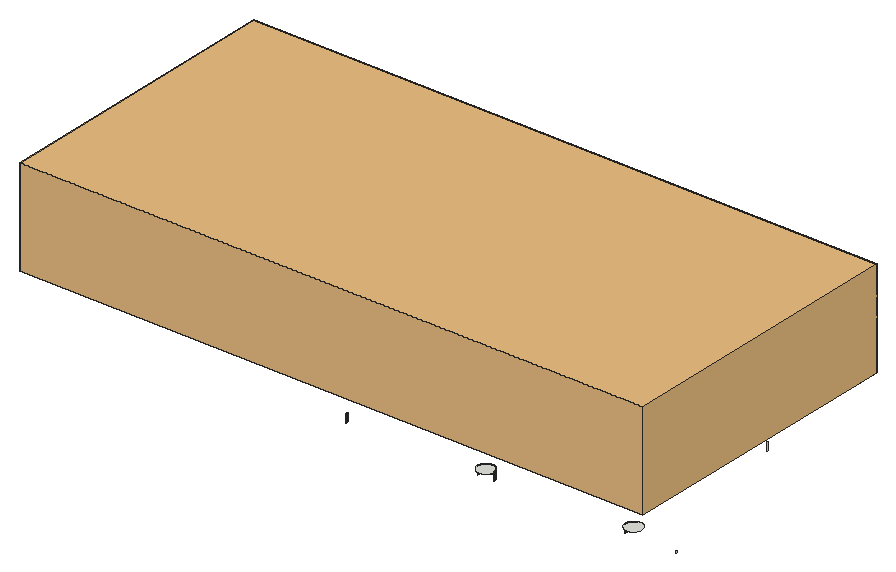
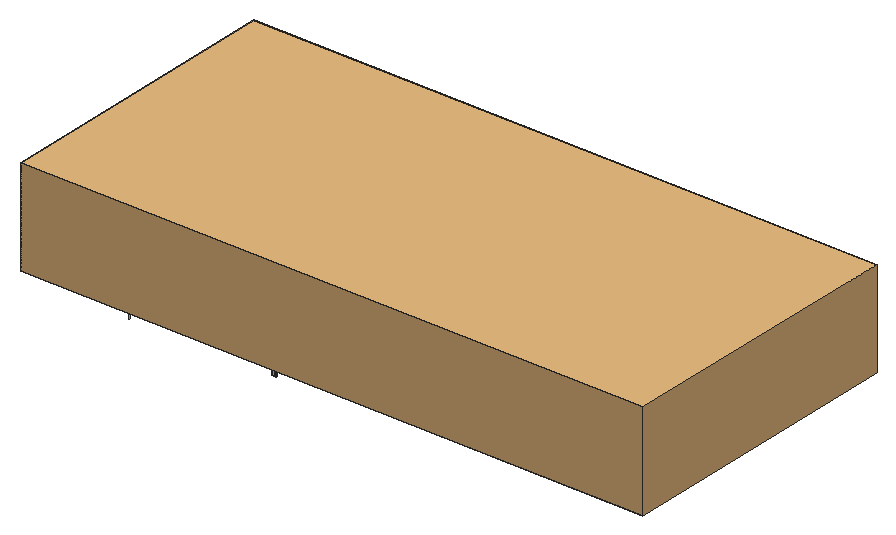
# SketchUp Ruby script. Lengths in inches.
U = 1.inch
M = Sketchup.active_model
def pt(a) = Geom::Point3d.new(a.map { |v| v * U })
def face(e, loops, mat)
  f = e.add_face(loops[0].map { |a| pt(a) })
  loops[1..].each { |l| e.add_face(l.map { |a| pt(a) }).erase! }
  f.material = f.back_material = mat if mat
  f
end
# faces: each face lists its corners as indices into pts; further lists are holes
def faces(e, pts, list, mat = nil) = list.each { |f| face(e, (f[0].is_a?(Array) ? f : [f]).map { |l| l.map { |i| pts[i] } }, mat) }
# xy, xz, yz: faces in a plane at the given z, y or x. An outline is a flat list of corners, or four numbers for a rectangle; further outlines are holes
def ring(l) = l.size == 4 ? [[l[0], l[1]], [l[2], l[1]], [l[2], l[3]], [l[0], l[3]]] : l.each_slice(2).to_a
def flat(e, list, mat, &to3) = list.each { |f| face(e, (f[0].is_a?(Array) ? f : [f]).map { |l| ring(l).map { |u, v| to3.(u, v) } }, mat) }
def xy(e, z, list, mat = nil) = flat(e, list, mat) { |x, y| [x, y, z] }
def xz(e, y, list, mat = nil) = flat(e, list, mat) { |x, z| [x, y, z] }
def yz(e, x, list, mat = nil) = flat(e, list, mat) { |y, z| [x, y, z] }
def lines(e, pts, list) = list.each { |a, b| e.add_line(pt(pts[a]), pt(pts[b])) }
# prism: a flat outline (further loops are holes) pulled along v
def prism(e, loops, v, mat = nil)
  f = face(e, loops, mat); d = Geom::Vector3d.new(v.map { |x| x * U })
  f.pushpull(f.normal.samedirection?(d) ? d.length : -d.length)
end
def box(e, o, s, mat = nil) = prism(e, [[o, [o[0] + s[0], o[1], o[2]], [o[0] + s[0], o[1] + s[1], o[2]], [o[0], o[1] + s[1], o[2]]]], [0, 0, s[2]], mat)
def at(x, y, z, deg = 0) = Geom::Transformation.translation(pt([x, y, z])) * Geom::Transformation.rotation(ORIGIN, Z_AXIS, deg.degrees)
def axes(o, x, y, z) = Geom::Transformation.new([*x, 0, *y, 0, *z, 0, *pt(o).to_a, 1])
def part(name) = M.definitions.add(name)
# library, detail: a bought-in or finely detailed component or shape, given as its bounding box
def library(name, o, s) = part(name).tap { |d| box(d.entities, o, s) }
def detail(e, o, s) = box(e.add_group.entities, o, s)
def put(e, d, t, mat = nil) = e.add_instance(d, t).tap { |i| i.material = mat if mat }
def group(e, t, mat = nil) = e.add_group.tap { |g| g.transformation = t; g.material = mat if mat }.entities
root = M.entities
M.materials.add("[Steel Brushed Stainless]1").color = [76, 76, 76]
c1 = library("Group\#19",[-3,0,0],[231,108,36])
xy(root,234,[[269.08,185,269,185.01,268.92,185.01,268.76,185.03,268.6875,185.04,268.61,185.06,268.53,185.08,268.46,185.09,268.38,185.11,268.3,185.14,268.23,185.16,268.16,185.1875,268.08,185.22,268.01,185.25,267.9375,185.28,267.87,185.3125,267.8,185.35,267.73,185.39,267.66,185.42,267.59,185.47,267.53,185.51,267.46,185.55,267.16,185.8,266.99,185.97,266.79,186.21,266.75,186.27,266.7,186.34,266.66,186.4,266.54,186.61,266.51,186.68,266.47,186.75,266.41,186.89,266.38,186.97,266.36,187.04,266.33,187.12,266.3125,187.19,266.29,187.27,266.27,187.34,266.26,187.42,266.24,187.5,266.23,187.58,266.22,187.65,266.21,187.73,266.21,187.81,266.2,187.89,266.2,188.125,266.21,188.2,266.21,188.28,266.22,188.36,266.23,188.4375,266.24,188.51,266.28,188.67,266.29,188.74,266.3125,188.82,266.34,188.9,266.36,188.97,266.39,189.04,266.42,189.12,266.51,189.33,266.59,189.47,266.625,189.54,266.67,189.61,266.71,189.67,266.75,189.74,267,190.04,267.17,190.21,267.41,190.41,267.47,190.45,267.54,190.5,267.6,190.54,267.81,190.66,267.88,190.69,267.95,190.73,268.09,190.79,268.17,190.82,268.24,190.84,268.32,190.87,268.39,190.89,268.47,190.91,268.54,190.93,268.62,190.94,268.7,190.96,268.78,190.97,268.85,190.98,268.93,190.99,269.01,190.99,269.09,191,269.32,191,269.4,190.99,269.48,190.99,269.64,190.97,269.71,190.96,269.87,190.92,269.94,190.91,270.02,190.89,270.1,190.86,270.17,190.84,270.24,190.8125,270.32,190.78,270.46,190.72,270.53,190.6875,270.6,190.65,270.67,190.61,270.74,190.58,270.81,190.53,270.87,190.49,270.9375,190.45,271.0625,190.35,271.12,190.3,271.24,190.2,271.41,190.03,271.61,189.79,271.65,189.73,271.7,189.66,271.74,189.6,271.86,189.39,271.89,189.32,271.93,189.25,271.99,189.11,272.02,189.03,272.04,188.96,272.07,188.88,272.09,188.81,272.11,188.73,272.13,188.66,272.14,188.58,272.16,188.5,272.17,188.42,272.18,188.35,272.1875,188.27,272.19,188.19,272.2,188.11,272.2,187.875,272.19,187.8,272.1875,187.72,272.18,187.64,272.17,187.5625,272.16,187.49,272.14,187.41,272.125,187.33,272.11,187.26,272.09,187.18,272.0625,187.1,272.04,187.03,272.01,186.96,271.98,186.88,271.89,186.67,271.81,186.53,271.78,186.46,271.73,186.39,271.69,186.33,271.65,186.26,271.4,185.96,271.23,185.79,270.99,185.59,270.93,185.55,270.86,185.5,270.8,185.46,270.59,185.34,270.52,185.31,270.45,185.27,270.31,185.21,270.23,185.18,270.16,185.16,270.08,185.13,270.01,185.11,269.93,185.09,269.86,185.07,269.78,185.06,269.7,185.04,269.55,185.02,269.47,185.01,269.39,185.01,269.3125,185],[323.875,185,323.8,185.01,323.72,185.01,323.64,185.02,323.5625,185.03,323.49,185.04,323.33,185.08,323.26,185.09,323.18,185.11,323.1,185.14,323.03,185.16,322.96,185.1875,322.88,185.22,322.74,185.28,322.67,185.3125,322.6,185.35,322.53,185.39,322.46,185.42,322.39,185.47,322.33,185.51,322.26,185.55,321.96,185.8,321.79,185.97,321.59,186.21,321.55,186.27,321.5,186.34,321.46,186.4,321.34,186.61,321.31,186.68,321.27,186.75,321.21,186.89,321.18,186.97,321.16,187.04,321.13,187.12,321.11,187.19,321.09,187.27,321.07,187.34,321.06,187.42,321.04,187.5,321.03,187.58,321.02,187.65,321.01,187.73,321.01,187.81,321,187.89,321,188.125,321.01,188.2,321.01,188.28,321.02,188.36,321.03,188.4375,321.04,188.51,321.08,188.67,321.09,188.74,321.11,188.82,321.14,188.9,321.16,188.97,321.1875,189.04,321.22,189.12,321.28,189.26,321.3125,189.33,321.35,189.4,321.39,189.47,321.42,189.54,321.47,189.61,321.51,189.67,321.55,189.74,321.8,190.04,321.97,190.21,322.21,190.41,322.27,190.45,322.34,190.5,322.4,190.54,322.61,190.66,322.68,190.69,322.75,190.73,322.89,190.79,322.97,190.82,323.04,190.84,323.12,190.87,323.19,190.89,323.27,190.91,323.34,190.93,323.42,190.94,323.5,190.96,323.58,190.97,323.65,190.98,323.73,190.99,323.81,190.99,323.89,191,324.125,191,324.2,190.99,324.28,190.99,324.36,190.98,324.4375,190.97,324.51,190.96,324.67,190.92,324.74,190.91,324.82,190.89,324.9,190.86,324.97,190.84,325.04,190.8125,325.12,190.78,325.26,190.72,325.33,190.6875,325.4,190.65,325.47,190.61,325.54,190.58,325.61,190.53,325.67,190.49,325.74,190.45,326.04,190.2,326.21,190.03,326.41,189.79,326.45,189.73,326.5,189.66,326.54,189.6,326.66,189.39,326.69,189.32,326.73,189.25,326.79,189.11,326.82,189.03,326.84,188.96,326.87,188.88,326.89,188.81,326.91,188.73,326.93,188.66,326.94,188.58,326.96,188.5,326.97,188.42,326.98,188.35,326.99,188.27,326.99,188.19,327,188.11,327,187.875,326.99,187.8,326.99,187.72,326.98,187.64,326.97,187.5625,326.96,187.49,326.92,187.33,326.91,187.26,326.89,187.18,326.86,187.1,326.84,187.03,326.8125,186.96,326.78,186.88,326.72,186.74,326.6875,186.67,326.65,186.6,326.61,186.53,326.58,186.46,326.53,186.39,326.49,186.33,326.45,186.26,326.2,185.96,326.03,185.79,325.79,185.59,325.73,185.55,325.66,185.5,325.6,185.46,325.39,185.34,325.32,185.31,325.25,185.27,325.11,185.21,325.03,185.18,324.96,185.16,324.88,185.13,324.81,185.11,324.73,185.09,324.66,185.07,324.58,185.06,324.5,185.04,324.42,185.03,324.35,185.02,324.27,185.01,324.19,185.01,324.11,185]])
xz(root,190.99,[[268.93,231,269.01,234],[269.4,231,269.48,234]])
xz(root,191,[[269.09,231,269.17,234],[269.17,231,269.25,234],[269.25,231,269.32,234]])
xz(root,251,[[269.08,231,269.15,234],[269.15,231,269.23,234],[269.23,231,269.3125,234]])
xz(root,251.01,[[268.92,231,269,234],[269.39,231,269.47,234]])
yz(root,217.39,[[188.19,231,188.27,234]])
yz(root,217.4,[[187.875,231,187.95,234],[187.95,231,188.03,234],[188.03,231,188.11,234]])
yz(root,266.2,[[187.89,231,187.97,234],[187.97,231,188.05,234],[188.05,231,188.125,234]])
yz(root,266.21,[[188.2,231,188.28,234]])
yz(root,272.2,[[187.875,231,187.95,234],[187.95,231,188.03,234],[188.03,231,188.11,234]])
yz(root,321,[[187.89,231,187.97,234],[187.97,231,188.05,234],[188.05,231,188.125,234]])
yz(root,321.01,[[188.2,231,188.28,234]])
yz(root,340,[[187.79,231,188,231.5]])
p = [[217.39,188.19,231],[217.4,188.11,231],[217.4,188.11,234],[217.39,188.19,234],[266.2,188.125,231],[266.21,188.2,231],
  [266.21,188.2,234],[266.2,188.125,234],[272.19,188.19,231],[272.2,188.11,231],[272.2,188.11,234],[272.19,188.19,234],
  [321,188.125,231],[321.01,188.2,231],[321.01,188.2,234],[321,188.125,234],[272.1875,188.27,231],[272.1875,188.27,234],
  [217.37,188.42,231],[217.38,188.35,231],[217.38,188.35,234],[217.37,188.42,234],[217.39,188.27,231],[217.39,188.27,234],
  [266.21,188.28,231],[266.22,188.36,231],[266.22,188.36,234],[266.21,188.28,234],[272.17,188.42,231],[272.18,188.35,231],
  [272.18,188.35,234],[272.17,188.42,234],[321.01,188.28,231],[321.02,188.36,231],[321.02,188.36,234],[321.01,188.28,234],
  [217.36,188.5,231],[217.36,188.5,234],[266.23,188.4375,231],[266.23,188.4375,234],[266.24,188.51,231],[266.24,188.51,234],
  [272.16,188.5,231],[272.16,188.5,234],[321.03,188.4375,231],[321.03,188.4375,234],[321.04,188.51,231],[321.04,188.51,234],
  [217.34,188.58,231],[217.34,188.58,234],[266.26,188.59,231],[266.26,188.59,234],[272.14,188.58,231],[272.14,188.58,234],
  [321.06,188.59,231],[321.06,188.59,234],[217.33,188.66,231],[217.33,188.66,234],[266.28,188.67,231],[266.28,188.67,234],
  [272.13,188.66,231],[272.13,188.66,234],[321.08,188.67,231],[321.08,188.67,234],[217.29,188.81,231],[217.31,188.73,231],
  [217.31,188.73,234],[217.29,188.81,234],[266.29,188.74,231],[266.29,188.74,234],[266.3125,188.82,231],[266.3125,188.82,234],
  [272.09,188.81,231],[272.11,188.73,231],[272.11,188.73,234],[272.09,188.81,234],[321.09,188.74,231],[321.09,188.74,234],
  [321.11,188.82,231],[321.11,188.82,234],[217.27,188.88,231],[217.27,188.88,234],[266.34,188.9,231],[266.34,188.9,234],
  [272.07,188.88,231],[272.07,188.88,234],[321.14,188.9,231],[321.14,188.9,234],[266.36,188.97,231],[266.36,188.97,234],
  [272.04,188.96,231],[272.04,188.96,234],[321.16,188.97,231],[321.16,188.97,234],[266.39,189.04,231],[266.39,189.04,234],
  [266.42,189.12,231],[266.42,189.12,234],[271.99,189.11,231],[272.02,189.03,231],[272.02,189.03,234],[271.99,189.11,234],
  [321.1875,189.04,231],[321.1875,189.04,234],[321.22,189.12,231],[321.22,189.12,234],[266.45,189.19,231],[266.45,189.19,234],
  [271.96,189.18,231],[271.96,189.18,234],[321.25,189.19,231],[321.25,189.19,234],[266.48,189.26,231],[266.48,189.26,234],
  [271.93,189.25,231],[271.93,189.25,234],[321.28,189.26,231],[321.28,189.26,234],[266.51,189.33,231],[266.51,189.33,234],
  [266.55,189.4,231],[266.55,189.4,234],[271.86,189.39,231],[271.89,189.32,231],[271.89,189.32,234],[271.86,189.39,234],
  [321.3125,189.33,231],[321.3125,189.33,234],[321.35,189.4,231],[321.35,189.4,234],[266.59,189.47,231],[266.59,189.47,234],
  [271.82,189.46,231],[271.82,189.46,234],[321.39,189.47,231],[321.39,189.47,234],[266.625,189.54,231],[266.625,189.54,234],
  [266.67,189.61,231],[266.67,189.61,234],[271.74,189.6,231],[271.78,189.53,231],[271.78,189.53,234],[271.74,189.6,234],
  [321.42,189.54,231],[321.42,189.54,234],[321.47,189.61,231],[321.47,189.61,234],[266.71,189.67,231],[266.71,189.67,234],
  [271.7,189.66,231],[271.7,189.66,234],[321.51,189.67,231],[321.51,189.67,234],[266.75,189.74,231],[266.75,189.74,234],
  [266.8,189.8,231],[266.8,189.8,234],[271.61,189.79,231],[271.65,189.73,231],[271.65,189.73,234],[271.61,189.79,234],
  [321.55,189.74,231],[321.55,189.74,234],[321.6,189.8,231],[321.6,189.8,234],[266.85,189.86,231],[266.85,189.86,234],
  [271.56,189.85,231],[271.56,189.85,234],[321.65,189.86,231],[321.65,189.86,234],[266.9,189.92,231],[266.9,189.92,234],
  [266.95,189.98,231],[266.95,189.98,234],[271.46,189.97,231],[271.51,189.91,231],[271.51,189.91,234],[271.46,189.97,234],
  [321.7,189.92,231],[321.7,189.92,234],[321.75,189.98,231],[321.75,189.98,234],[267,190.04,231],[267,190.04,234],
  [267.06,190.1,231],[267.06,190.1,234],[271.35,190.09,231],[271.41,190.03,231],[271.41,190.03,234],[271.35,190.09,234],
  [321.8,190.04,231],[321.8,190.04,234],[321.86,190.1,231],[321.86,190.1,234],[267.11,190.15,231],[267.11,190.15,234],
  [271.24,190.2,231],[271.3,190.14,231],[271.3,190.14,234],[271.24,190.2,234],[321.91,190.15,231],[321.91,190.15,234],
  [267.17,190.21,231],[267.17,190.21,234],[267.23,190.26,231],[267.23,190.26,234],[271.18,190.25,231],[271.18,190.25,234],
  [321.97,190.21,231],[321.97,190.21,234],[322.03,190.26,231],[322.03,190.26,234],[267.29,190.31,231],[267.29,190.31,234],
  [267.35,190.36,231],[267.35,190.36,234],[271.0625,190.35,231],[271.12,190.3,231],[271.12,190.3,234],[271.0625,190.35,234],
  [322.09,190.31,231],[322.09,190.31,234],[322.15,190.36,231],[322.15,190.36,234],[267.41,190.41,231],[267.41,190.41,234],
  [267.47,190.45,231],[267.47,190.45,234],[270.87,190.49,231],[270.9375,190.45,231],[270.9375,190.45,234],[270.87,190.49,234],
  [271,190.4,231],[271,190.4,234],[322.21,190.41,231],[322.21,190.41,234],[322.27,190.45,231],[322.27,190.45,234],
  [267.54,190.5,231],[267.54,190.5,234],[267.6,190.54,231],[267.6,190.54,234],[267.67,190.58,231],[267.67,190.58,234],
  [270.74,190.58,231],[270.81,190.53,231],[270.81,190.53,234],[270.74,190.58,234],[322.34,190.5,231],[322.34,190.5,234],
  [322.4,190.54,231],[322.4,190.54,234],[322.47,190.58,231],[322.47,190.58,234],[267.74,190.62,231],[267.74,190.62,234],
  [267.81,190.66,231],[267.81,190.66,234],[270.6,190.65,231],[270.67,190.61,231],[270.67,190.61,234],[270.6,190.65,234],
  [322.54,190.62,231],[322.54,190.62,234],[322.61,190.66,231],[322.61,190.66,234],[267.88,190.69,231],[267.88,190.69,234],
  [267.95,190.73,231],[267.95,190.73,234],[268.02,190.76,231],[268.02,190.76,234],[270.39,190.75,231],[270.46,190.72,231],
  [270.46,190.72,234],[270.39,190.75,234],[270.53,190.6875,231],[270.53,190.6875,234],[322.68,190.69,231],[322.68,190.69,234],
  [322.75,190.73,231],[322.75,190.73,234],[322.82,190.76,231],[322.82,190.76,234],[268.09,190.79,231],[268.09,190.79,234],
  [268.17,190.82,231],[268.17,190.82,234],[268.24,190.84,231],[268.24,190.84,234],[268.32,190.87,231],[268.32,190.87,234],
  [270.1,190.86,231],[270.17,190.84,231],[270.17,190.84,234],[270.1,190.86,234],[270.24,190.8125,231],[270.24,190.8125,234],
  [270.32,190.78,231],[270.32,190.78,234],[322.89,190.79,231],[322.89,190.79,234],[322.97,190.82,231],[322.97,190.82,234],
  [323.04,190.84,231],[323.04,190.84,234],[323.12,190.87,231],[323.12,190.87,234],[268.39,190.89,231],[268.39,190.89,234],
  [268.47,190.91,231],[268.47,190.91,234],[268.54,190.93,231],[268.54,190.93,234],[268.62,190.94,231],[268.62,190.94,234],
  [268.7,190.96,231],[268.7,190.96,234],[269.71,190.96,231],[269.79,190.94,231],[269.79,190.94,234],[269.71,190.96,234],
  [269.87,190.92,231],[269.87,190.92,234],[269.94,190.91,231],[269.94,190.91,234],[270.02,190.89,231],[270.02,190.89,234],
  [268.78,190.97,231],[268.78,190.97,234],[268.85,190.98,231],[268.85,190.98,234],[268.93,190.99,231],[268.93,190.99,234],
  [269.01,190.99,231],[269.09,191,231],[269.09,191,234],[269.01,190.99,234],[269.32,191,231],[269.4,190.99,231],
  [269.4,190.99,234],[269.32,191,234],[269.48,190.99,231],[269.56,190.98,231],[269.56,190.98,234],[269.48,190.99,234],
  [269.64,190.97,231],[269.64,190.97,234],[268.6875,251.04,231],[268.61,251.06,231],[268.61,251.06,234],[268.6875,251.04,234],
  [268.76,251.03,231],[268.76,251.03,234],[268.84,251.02,231],[268.84,251.02,234],[268.92,251.01,231],[268.92,251.01,234],
  [269.08,251,231],[269,251.01,231],[269,251.01,234],[269.08,251,234],[269.39,251.01,231],[269.3125,251,231],
  [269.3125,251,234],[269.39,251.01,234],[269.55,251.02,231],[269.47,251.01,231],[269.47,251.01,234],[269.55,251.02,234],
  [269.625,251.03,231],[269.625,251.03,234],[269.7,251.04,231],[269.7,251.04,234],[269.78,251.06,231],[269.78,251.06,234],
  [268.38,251.11,231],[268.3,251.14,231],[268.3,251.14,234],[268.38,251.11,234],[268.46,251.09,231],[268.46,251.09,234],
  [268.53,251.08,231],[268.53,251.08,234],[269.86,251.07,231],[269.86,251.07,234],[269.93,251.09,231],[269.93,251.09,234],
  [270.01,251.11,231],[270.01,251.11,234],[270.08,251.13,231],[270.08,251.13,234],[270.16,251.16,231],[270.16,251.16,234],
  [323.1,251.14,231],[323.03,251.16,231],[323.03,251.16,234],[323.1,251.14,234]]
faces(root,p,[[0,1,2,3],[4,5,6,7],[8,9,10,11],[12,13,14,15],[16,8,11,17],[18,19,20,21],[19,22,23,20],[24,25,26,27],
  [28,29,30,31],[29,16,17,30],[32,33,34,35],[36,18,21,37],[25,38,39,26],[38,40,41,39],[42,28,31,43],[33,44,45,34],
  [44,46,47,45],[48,36,37,49],[40,50,51,41],[52,42,43,53],[46,54,55,47],[56,48,49,57],[50,58,59,51],[60,52,53,61],
  [54,62,63,55],[64,65,66,67],[65,56,57,66],[58,68,69,59],[68,70,71,69],[72,73,74,75],[73,60,61,74],[62,76,77,63],
  [76,78,79,77],[80,64,67,81],[70,82,83,71],[84,72,75,85],[78,86,87,79],[82,88,89,83],[90,84,85,91],[86,92,93,87],
  [88,94,95,89],[94,96,97,95],[98,99,100,101],[99,90,91,100],[92,102,103,93],[102,104,105,103],[96,106,107,97],[108,98,101,109],
  [104,110,111,105],[106,112,113,107],[114,108,109,115],[110,116,117,111],[112,118,119,113],[118,120,121,119],[122,123,124,125],[123,114,115,124],
  [116,126,127,117],[126,128,129,127],[120,130,131,121],[132,122,125,133],[128,134,135,129],[130,136,137,131],[136,138,139,137],[140,141,142,143],
  [141,132,133,142],[134,144,145,135],[144,146,147,145],[138,148,149,139],[150,140,143,151],[146,152,153,147],[148,154,155,149],[154,156,157,155],
  [158,159,160,161],[159,150,151,160],[152,162,163,153],[162,164,165,163],[156,166,167,157],[168,158,161,169],[164,170,171,165],[166,172,173,167],
  [172,174,175,173],[176,177,178,179],[177,168,169,178],[170,180,181,171],[180,182,183,181],[174,184,185,175],[184,186,187,185],[188,189,190,191],
  [189,176,179,190],[182,192,193,183],[192,194,195,193],[186,196,197,187],[198,199,200,201],[199,188,191,200],[194,202,203,195],[196,204,205,197],
  [204,206,207,205],[208,198,201,209],[202,210,211,203],[210,212,213,211],[206,214,215,207],[214,216,217,215],[218,219,220,221],[219,208,209,220],
  [212,222,223,213],[222,224,225,223],[216,226,227,217],[226,228,229,227],[230,231,232,233],[231,234,235,232],[234,218,221,235],[224,236,237,225],
  [236,238,239,237],[228,240,241,229],[240,242,243,241],[242,244,245,243],[246,247,248,249],[247,230,233,248],[238,250,251,239],[250,252,253,251],
  [252,254,255,253],[244,256,257,245],[256,258,259,257],[260,261,262,263],[261,246,249,262],[254,264,265,255],[264,266,267,265],[258,268,269,259],
  [268,270,271,269],[270,272,273,271],[274,275,276,277],[275,278,279,276],[278,260,263,279],[266,280,281,267],[280,282,283,281],[282,284,285,283],
  [272,286,287,273],[286,288,289,287],[288,290,291,289],[290,292,293,291],[294,295,296,297],[295,298,299,296],[298,300,301,299],[300,274,277,301],
  [284,302,303,285],[302,304,305,303],[304,306,307,305],[306,308,309,307],[292,310,311,293],[310,312,313,311],[312,314,315,313],[314,316,317,315],
  [316,318,319,317],[320,321,322,323],[321,324,325,322],[324,326,327,325],[326,328,329,327],[328,294,297,329],[318,330,331,319],[330,332,333,331],
  [332,334,335,333],[336,337,338,339],[340,341,342,343],[344,345,346,347],[345,348,349,346],[348,320,323,349],[350,351,352,353],[354,350,353,355],
  [356,354,355,357],[358,356,357,359],[360,361,362,363],[364,365,366,367],[368,369,370,371],[372,368,371,373],[374,372,373,375],[376,374,375,377],
  [378,379,380,381],[382,378,381,383],[384,382,383,385],[351,384,385,352],[386,376,377,387],[388,386,387,389],[390,388,389,391],[392,390,391,393],
  [394,392,393,395],[396,397,398,399]])
put(root,c1,at(114,170,252),"[Steel Brushed Stainless]1")
